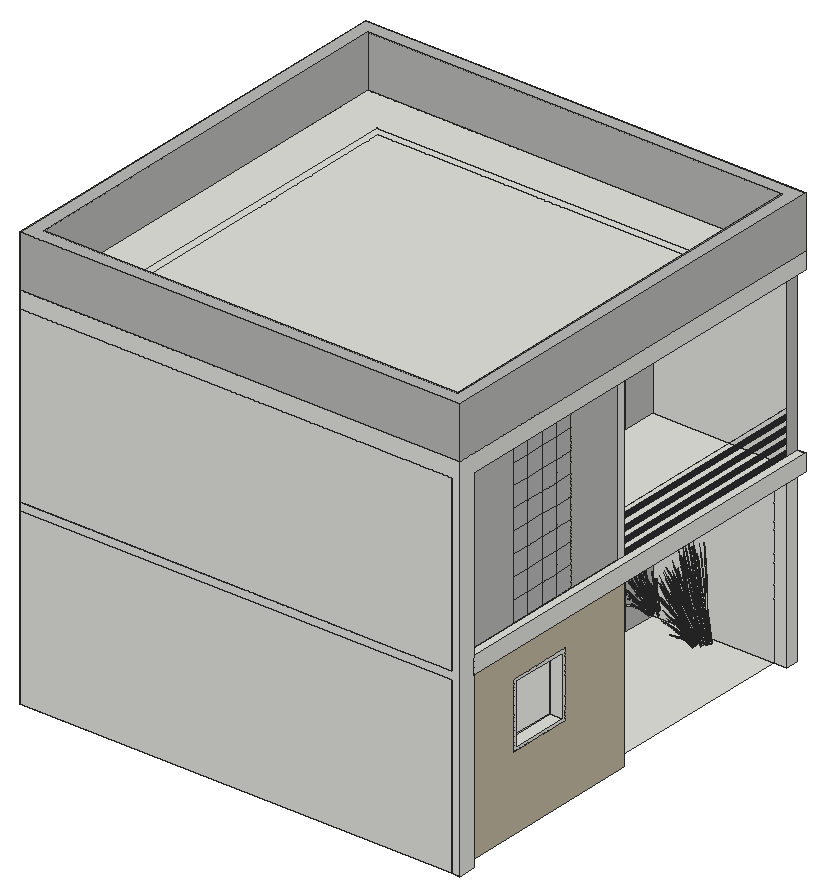
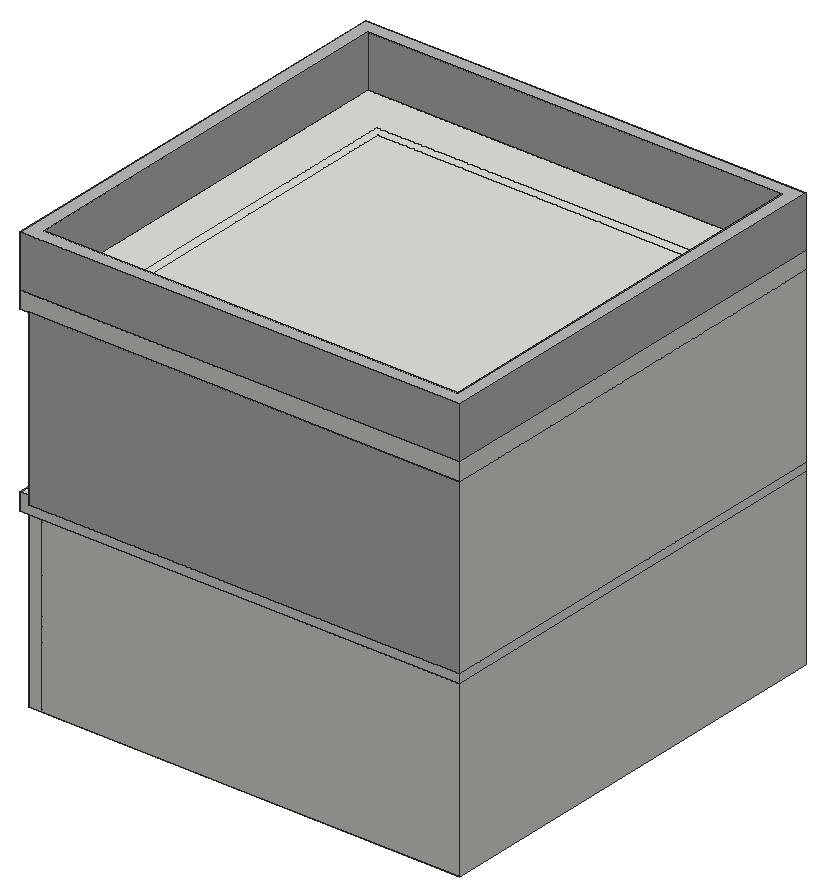
# SketchUp Ruby script. Lengths in inches.
U = 1.inch
M = Sketchup.active_model
def pt(a) = Geom::Point3d.new(a.map { |v| v * U })
def face(e, loops, mat)
  f = e.add_face(loops[0].map { |a| pt(a) })
  loops[1..].each { |l| e.add_face(l.map { |a| pt(a) }).erase! }
  f.material = f.back_material = mat if mat
  f
end
# faces: each face lists its corners as indices into pts; further lists are holes
def faces(e, pts, list, mat = nil) = list.each { |f| face(e, (f[0].is_a?(Array) ? f : [f]).map { |l| l.map { |i| pts[i] } }, mat) }
# xy, xz, yz: faces in a plane at the given z, y or x. An outline is a flat list of corners, or four numbers for a rectangle; further outlines are holes
def ring(l) = l.size == 4 ? [[l[0], l[1]], [l[2], l[1]], [l[2], l[3]], [l[0], l[3]]] : l.each_slice(2).to_a
def flat(e, list, mat, &to3) = list.each { |f| face(e, (f[0].is_a?(Array) ? f : [f]).map { |l| ring(l).map { |u, v| to3.(u, v) } }, mat) }
def xy(e, z, list, mat = nil) = flat(e, list, mat) { |x, y| [x, y, z] }
def xz(e, y, list, mat = nil) = flat(e, list, mat) { |x, z| [x, y, z] }
def yz(e, x, list, mat = nil) = flat(e, list, mat) { |y, z| [x, y, z] }
def lines(e, pts, list) = list.each { |a, b| e.add_line(pt(pts[a]), pt(pts[b])) }
# prism: a flat outline (further loops are holes) pulled along v
def prism(e, loops, v, mat = nil)
  f = face(e, loops, mat); d = Geom::Vector3d.new(v.map { |x| x * U })
  f.pushpull(f.normal.samedirection?(d) ? d.length : -d.length)
end
def box(e, o, s, mat = nil) = prism(e, [[o, [o[0] + s[0], o[1], o[2]], [o[0] + s[0], o[1] + s[1], o[2]], [o[0], o[1] + s[1], o[2]]]], [0, 0, s[2]], mat)
def at(x, y, z, deg = 0) = Geom::Transformation.translation(pt([x, y, z])) * Geom::Transformation.rotation(ORIGIN, Z_AXIS, deg.degrees)
def axes(o, x, y, z) = Geom::Transformation.new([*x, 0, *y, 0, *z, 0, *pt(o).to_a, 1])
def part(name) = M.definitions.add(name)
# library, detail: a bought-in or finely detailed component or shape, given as its bounding box
def library(name, o, s) = part(name).tap { |d| box(d.entities, o, s) }
def detail(e, o, s) = box(e.add_group.entities, o, s)
def put(e, d, t, mat = nil) = e.add_instance(d, t).tap { |i| i.material = mat if mat }
def group(e, t, mat = nil) = e.add_group.tap { |g| g.transformation = t; g.material = mat if mat }.entities
root = M.entities
M.materials.add("Brick_05_1K").color = [195, 185, 161]
M.materials.add("Glass_Basic_01").color = [161, 173, 186]
M.materials["Glass_Basic_01"].alpha = 0.25
M.materials.add("Glass_Mirror_01").color = [185, 185, 185]
M.materials.add("LightPink_Translucent").color = [144, 107, 117]
M.materials["LightPink_Translucent"].alpha = 0.75
M.materials.add("Plywood_01_1K").color = [125, 96, 64]
M.materials.add("ThomThom - Buttons1").color = [48, 49, 53]
M.materials.add("ThomThom - Waistcoat2").color = [186, 186, 184]
M.materials.add("Wood_Veneer_15_1K").color = [103, 69, 45]
c1 = part("blade")
p = [[2.15,0.21,22],[0,0.17,0],[0.09,0.45,0],[2.18,0.31,22],[2.29,0.31,22],[0.38,0.45,0],
  [2.48,0.24,33],[2.49,0.24,33],[2.48,0.22,33]]
faces(c1.entities,p,[[0,1,2,3],[4,5,2,3],[6,3,4,7],[8,0,3,6]])
c2 = part("blade with seeds\#1")
put(c2.entities,c1,at(0,0,0))
c3 = part("seeds")
p = [[0.3,-0.1,1.38],[-0.01,-0.03,1.59],[-0.01,-0.03,0.03],[0.14,-0.07,-0.07],[0.29,-0.03,3],[0.15,0.01,3.11]]
faces(c3.entities,p,[[0,1,2,3],[1,0,4,5]],"LightPink_Translucent")
c4 = part("blade with seeds")
put(c4.entities,c1,at(0,0,0))
put(c4.entities,c3,axes([2.4,0.25,30.99],[1.5799,-0.05474,1.17369],[-0.12525,1.92788,0.29478],[-0.07173,-0.02425,1.56792]))
g1 = group(root,at(0,0,0))
xy(g1,0,[[9,9,291,144],[9,150,291,291]])
g2 = group(g1,at(0,0,0))
xy(g2,0,[[[0,0,0,300,300,300,300,291,207,291,207,150,300,150,300,0],[9,9,291,9,291,144,9,144,9,150,201,150,201,291,9,291]]])
xy(g2,3,[[201,174,207,216],[201,222,207,264]])
xy(g2,53.72,[[291,55.83,300,96.48]])
xy(g2,81,[[201,174,207,216],[201,222,207,264]])
xy(g2,94.93,[[291,55.83,300,96.48]])
xz(g2,0,[[0,0,300,120]])
xz(g2,9,[[9,0,291,120]])
xz(g2,55.83,[[291,53.72,300,94.93]])
xz(g2,96.48,[[291,53.72,300,94.93]])
xz(g2,144,[[9,0,291,120]])
xz(g2,150,[[9,0,201,120],[207,0,300,120]])
xz(g2,174,[[201,3,207,81]])
xz(g2,216,[[201,3,207,81]])
xz(g2,222,[[201,3,207,81]])
xz(g2,264,[[201,3,207,81]])
xz(g2,291,[[9,0,201,120],[201,0,207,120],[207,0,291,120],[291,0,300,120]])
xz(g2,300,[[0,0,291,120],[291,0,300,120]])
yz(g2,0,[[0,0,300,120]])
yz(g2,9,[[9,0,144,120],[144,0,150,120],[150,0,291,120]])
yz(g2,201,[[[150,0,291,120],[222,3,264,81],[174,3,216,81]]])
yz(g2,201,[[174,3,216,81],[222,3,264,81]],"Glass_Basic_01")
yz(g2,207,[[150,0,171,0,171,84,267,84,267,0,291,0,291,120,150,120]],"ThomThom - Waistcoat2")
yz(g2,207,[[[171,0,219,84],[174,3,216,81]],[[219,0,267,84],[222,3,264,81]]],"Wood_Veneer_15_1K")
yz(g2,291,[[[9,0,144,120],[55.83,53.72,96.48,94.93]]])
yz(g2,300,[[291,0,300,120],[[53.83,51.72,98.48,96.93],[55.83,53.72,96.48,94.93]]])
yz(g2,300,[[[0,0,150,120],[53.83,51.72,98.48,96.93]]],"Brick_05_1K")
p = [[207,150,126],[207,150,120]]
lines(g2,p,[[0,1]])
g3 = group(g1,at(0,0,120))
xy(g3,-120,[[300,0,306,12]])
xy(g3,0,[[0,0,0,300,306,300,306,12,300,12,300,0]])
xy(g3,6,[[0,0,300,300]])
xy(g3,12,[[300,12,306,300]])
xy(g3,126,[[0,0,300,12],[0,12,306,300]])
xy(g3,138,[[[9,9,297,291],[39,39,267,261]],[[39,39,267,261],[45,45,261,255]],[45,45,261,255]])
xz(g3,0,[[300,-120,306,-120,306,138,0,138,0,126,300,126,300,6,0,6,0,0,300,0]])
xz(g3,12,[[300,-120,306,0],[300,12,306,126]])
xz(g3,300,[[0,0,0,6,300,6,300,12,306,12,306,0],[0,126,306,138]])
yz(g3,0,[[0,0,300,6],[0,126,300,138]])
yz(g3,300,[[0,-120,12,0],[0,6,0,126,12,126,12,12,300,12,300,6]])
yz(g3,306,[[0,-120,12,-120,12,126,300,126,300,138,0,138],[12,0,300,12]])
g4 = group(g3,at(0,0,138),"ThomThom - Waistcoat2")
prism(g4,[[[306,300,0],[306,0,0],[0,0,0],[0,300,0]],[[297,291,0],[9,291,0],[9,9,0],[297,9,0]]],[0,0,36])
g5 = group(g1,at(0,0,126))
xy(g5,0,[[[0,0,0,300,300,300,300,291,207,291,207,150,201,150,201,291,9,291,9,9,201,9,201,144,9,144,9,150,300,150,300,0],[207,9,291,144]]])
xy(g5,3,[[201,174,207,216],[201,222,207,264]])
xy(g5,81,[[201,174,207,216],[201,222,207,264]])
xy(g5,120,[[[0,0,300,0,300,144,291,144,291,9,207,9,207,291,300,291,300,300,0,300],[9,9,9,291,201,291,201,150,9,150,9,144,201,144,201,9]],[207,144,300,150]])
xz(g5,0,[[0,0,300,120]])
xz(g5,9,[[9,0,201,120],[201,0,207,120],[207,0,291,120]])
xz(g5,144,[[9,0,201,120],[207,0,291,120]])
xz(g5,150,[[9,0,201,120],[207,0,300,36]])
xz(g5,150,[[207,36,300,120]],"ThomThom - Waistcoat2")
xz(g5,174,[[201,3,207,81]])
xz(g5,216,[[201,3,207,81]])
xz(g5,222,[[201,3,207,81]])
xz(g5,264,[[201,3,207,81]])
xz(g5,291,[[9,0,201,120],[207,0,300,120]])
xz(g5,300,[[0,0,300,120]],"ThomThom - Waistcoat2")
yz(g5,0,[[0,0,300,120]])
yz(g5,9,[[9,0,144,120],[144,0,150,120],[150,0,291,120]])
yz(g5,201,[[9,0,144,120],[[150,0,291,120],[222,3,264,81],[174,3,216,81]]])
yz(g5,201,[[174,3,216,81],[222,3,264,81]],"Plywood_01_1K")
yz(g5,207,[[9,0,144,120],[[171,0,219,84],[174,3,216,81]],[[219,0,267,84],[222,3,264,81]]])
yz(g5,207,[[150,0,171,0,171,84,267,84,267,0,291,0,291,120,150,120]],"ThomThom - Waistcoat2")
yz(g5,291,[[9,0,144,120]])
yz(g5,300,[[144,0,150,120],[150,0,291,5.71]])
yz(g5,300,[[53.1875,6,65.8,20.25],[65.8,6,78.41,20.25],[78.41,6,91.03,20.25],[91.03,6,103.64,20.25],[53.1875,20.25,65.8,34.5],
  [65.8,20.25,78.41,34.5],[78.41,20.25,91.03,34.5],[91.03,20.25,103.64,34.5],[53.1875,34.5,65.8,48.75],[65.8,34.5,78.41,48.75],
  [78.41,34.5,91.03,48.75],[91.03,34.5,103.64,48.75],[53.1875,48.75,65.8,63],[65.8,48.75,78.41,63],[78.41,48.75,91.03,63],
  [91.03,48.75,103.64,63],[53.1875,63,65.8,77.25],[65.8,63,78.41,77.25],[78.41,63,91.03,77.25],[91.03,63,103.64,77.25],
  [53.1875,77.25,65.8,91.5],[65.8,77.25,78.41,91.5],[78.41,77.25,91.03,91.5],[91.03,77.25,103.64,91.5],[53.1875,91.5,65.8,105.75],
  [65.8,91.5,78.41,105.75],[78.41,91.5,91.03,105.75],[91.03,91.5,103.64,105.75],[53.1875,105.75,65.8,120],[65.8,105.75,78.41,120],
  [78.41,105.75,91.03,120],[91.03,105.75,103.64,120]],"Glass_Mirror_01")
yz(g5,300,[[150,5.71,291,9.5],[150,13.28,291,17.07],[150,20.86,291,24.64],[150,28.43,291,32.21]],"ThomThom - Buttons1")
yz(g5,300,[[0,0,144,0,144,120,103.64,120,103.64,6,53.1875,6,53.1875,120,0,120],[291,0,300,120]],"ThomThom - Waistcoat2")
p = [[300,150,36],[300,291,36]]
lines(g5,p,[[0,1]])
put(root,c2,axes([216.57,273.84,13.09],[-0.07697,0.17304,1.5897],[-0.85991,0.44448,-0.24285],[-0.23336,-0.29985,0.27078]))
put(root,c2,axes([218.64,273.875,15.96],[-0.89213,0.297,-0.46065],[-0.15606,-1.12475,-0.35681],[-0.23962,-0.32232,0.88141]))
put(root,c2,axes([219,273.85,16.23],[-0.77091,-0.6039,-0.64046],[0.54787,-1.05824,0.07729],[-0.27931,-0.36058,0.906]))
put(root,c2,axes([219.28,273.34,16.28],[-0.53874,1.06944,-0.10962],[-0.78019,-0.61612,-0.60845],[-0.2712,-0.30214,0.92453]))
put(root,c2,axes([218.29,272.97,14.08],[-0.02894,0.41302,1.28914],[-0.77632,0.42312,-0.27724],[-0.21961,-0.50739,0.55117]))
put(root,c2,axes([219.04,270.71,15.98],[-0.00742,0.151,1.59908],[-0.79509,0.62706,-0.1511],[-0.26143,-0.25182,0.28298]))
put(root,c2,axes([216.86,272.49,14.23],[0.49736,0.38508,1.03545],[-0.66822,0.331,0.76078],[-0.16744,-0.31805,0.22807]))
put(root,c2,axes([218.73,273.05,15.82],[-0.13963,-1.00636,-0.31925],[0.79822,-0.26574,0.41216],[-0.2144,-0.28839,0.78863]))
put(root,c2,axes([218.9,273.18,16.01],[0.89921,-0.28673,0.43274],[0.15606,1.12475,0.35681],[-0.21148,-0.33149,0.89544]))
put(root,c2,axes([219.08,272.95,16],[0.4109,-0.79368,0.05797],[0.58514,0.46209,0.45634],[-0.18917,-0.25446,0.69585]))
put(root,c2,axes([219.99,270.14,15.99],[-0.14882,-0.16043,1.57709],[-0.91289,0.20534,-0.24942],[-0.17308,-0.40254,0.12648]))
put(root,c2,axes([217,275.05,13.88],[-0.97904,-0.72283,0],[0.54599,-1.20931,-0.46523],[0.12435,-0.27543,1.47583]))
put(root,c2,axes([221.38,273.3,16.28],[-0.88471,0.5817,-0.10962],[-0.43476,-1.03242,-0.60845],[-0.11673,-0.43507,0.92453]))
put(root,c2,axes([220.62,273.35,15.96],[-0.88873,-0.31321,-0.46065],[0.30463,-1.07385,-0.35681],[-0.08149,-0.43235,0.88141]))
put(root,c2,axes([220.87,272.21,13.53],[0.11725,0.74462,1.27635],[-0.9333,0.11852,0.07306],[-0.14126,-0.52153,0.72629]))
put(root,c2,axes([220.04,270.85,13.78],[-0.62476,0.71677,-0.05849],[-0.57245,-0.78502,-0.26518],[-0.0403,-0.22243,0.87466]))
put(root,c2,axes([220.94,273.56,16.23],[-0.4315,-1.0159,-0.64046],[0.88824,-0.56616,0.07729],[-0.1009,-0.49086,0.906]))
put(root,c2,axes([221.11,273.71,16.29],[-0.27256,0.96081,0.31925],[-0.79518,-0.28024,-0.41216],[-0.07291,-0.38684,0.78863]))
put(root,c2,axes([220.26,271.39,13.09],[-0.14833,0.06042,1.5897],[-0.86768,-0.41907,-0.24285],[-0.01248,-0.42273,0.27078]))
put(root,c2,axes([217.59,274.39,13.56],[0.48852,-1.08202,-0.44759],[0.87598,0.64674,0],[0.11126,-0.24644,1.41987]))
put(root,c2,axes([221.02,272.69,15.82],[0.27256,-0.96081,-0.31925],[0.79518,0.28024,0.41216],[-0.07291,-0.38684,0.78863]))
put(root,c2,axes([220.04,275.3125,15.23],[0.02213,0.47954,1.54493],[-0.95907,-0.31812,0.12492],[0.05932,-0.68338,0.66044]))
put(root,c2,axes([221.36,272.84,16],[0.66618,-0.42462,0.05797],[0.32607,0.77431,0.45634],[-0.06434,-0.34133,0.69585]))
put(root,c2,axes([221.12,272.92,16.01],[0.89085,0.32663,0.43274],[-0.30463,1.07385,0.35681],[-0.05354,-0.4223,0.89544]))
put(root,c2,axes([221.1875,270.66,14.23],[0.1613,0.71432,1.03545],[-0.66662,-0.33623,0.76078],[0.04561,-0.37895,0.22807]))
put(root,c2,axes([219.46,275.97,13.6],[0.16018,-1.20264,-0.5621],[0.98808,0.25378,-0.14753],[0.11973,-0.3589,1.24074]))
put(root,c2,axes([224.01,270.99,15.98],[-0.08553,0.10454,1.59908],[-0.91687,-0.22868,-0.1511],[-0.05858,-0.41178,0.28298]))
put(root,c2,axes([223.24,271.9,15.28],[-0.82131,0.22128,-0.03148],[-0.18882,-1.04586,-0.14272],[0.05207,-0.2184,0.47074]))
put(root,c2,axes([223.22,274.61,16.28],[-0.99362,-0.0619,-0.10962],[0.02716,-1.17208,-0.60845],[0.06902,-0.45141,0.92453]))
put(root,c2,axes([222.83,274.79,16.29],[-0.61172,0.65782,0.31925],[-0.57907,-0.75112,-0.41216],[0.08811,-0.38163,0.78863]))
put(root,c2,axes([222.25,272,14.08],[-0.2403,0.27843,1.28914],[-0.79492,-0.36227,-0.27724],[0.10768,-0.56334,0.55117]))
put(root,c2,axes([222.62,273.59,15.99],[-0.01652,-0.24801,1.57709],[-0.75906,-0.68026,-0.24942],[0.1002,-0.44114,0.12648]))
put(root,c2,axes([222.74,274.55,16.23],[0.02352,-1.1557,-0.64046],[0.99061,0.07762,0.07729],[0.10454,-0.48961,0.906]))
put(root,c2,axes([223.15,273.86,15.82],[0.61172,-0.65782,-0.31925],[0.57907,0.75112,0.41216],[0.08811,-0.38163,0.78863]))
put(root,c2,axes([223.38,274.19,16],[0.74296,0.05822,0.05797],[-0.02037,0.87906,0.45634],[0.07774,-0.33673,0.69585]))
put(root,c2,axes([223.14,274.11,16.01],[0.64379,0.85247,0.43274],[-0.68369,0.73521,0.35681],[0.11875,-0.39995,0.89544]))
put(root,c2,axes([221.58,276.22,15.23],[-0.16834,0.42944,1.54493],[-0.70619,-0.88871,0.12492],[0.31858,-0.5539,0.66044]))
put(root,c2,axes([224.54,274.45,13.09],[-0.14106,-0.08423,1.5897],[-0.41543,-1.06044,-0.24285],[0.21501,-0.3215,0.27078]))
put(root,c2,axes([223.88,276.1,15.96],[-0.23225,-1.14083,-0.46065],[0.87956,-0.19957,-0.35681],[0.25205,-0.30642,0.88141]))
put(root,c4,axes([260.33,260.75,16.11],[0.50831,-0.02346,1.71376],[-0.33721,1.01661,0.13857],[-0.72439,-0.06288,0.73262]))
put(root,c4,axes([260.54,262.54,16.11],[0.42521,-0.21906,1.71376],[0.35798,1.01226,0.13857],[-0.66754,0.22878,0.73262]))
put(root,c4,axes([259.22,264.27,14.83],[0.42589,0.08502,1.43002],[0.2745,0.86839,-0.30754],[-0.57851,0.16255,0.61141]))
put(root,c4,axes([262.98,261.49,15.58],[0.34834,-0.14982,1.77064],[0.12012,1.04605,0.13857],[-0.75452,0.1388,0.63284]))
put(root,c4,axes([259.24,262.1875,16.95],[-0.20012,0.13446,1.74944],[0.01702,0.98243,-0.27667],[-0.45871,0.12776,0.14031]))
put(root,c4,axes([261.85,259.81,17.22],[-1.22504,-0.02494,-0.71045],[0.08228,-1.05005,0.08574],[-0.51899,-0.11081,1.00501]))
put(root,c4,axes([260.86,260.07,14.83],[0.23927,0.28834,1.43002],[-0.55135,0.78376,-0.30754],[-0.56612,-0.18733,0.61141]))
put(root,c4,axes([259.88,261.63,16.76],[-1.01846,-0.28891,-0.35414],[0.29705,-0.84289,0.4572],[-0.41005,0.07729,0.87481]))
put(root,c4,axes([261.29,259.125,16.11],[0.45521,0.17844,1.71376],[-0.94204,0.74856,0.13857],[-0.58713,-0.33769,0.73262]))
put(root,c4,axes([257.01,263.18,16.95],[0.1564,0.02778,1.77383],[0.48382,0.91506,-0.16761],[-0.32016,0.24017,0.31391]))
put(root,c4,axes([260.58,262.06,16.92],[-0.332,0.94205,-0.51099],[-1.13828,-0.3229,-0.3958],[-0.45829,0.08638,0.97773]))
put(root,c4,axes([261.44,260.02,16.92],[-0.88986,0.68603,-0.51099],[-0.77932,-0.72471,-0.3958],[-0.45212,-0.10438,0.97773]))
put(root,c4,axes([260.01,262,13.73],[0.03108,0.16322,1.76342],[-0.62654,0.85237,-0.26939],[-0.44504,-0.04296,0.30037]))
put(root,c4,axes([260.1875,258.1,16.95],[0.09085,0.10335,1.77383],[-0.43798,0.92907,-0.16761],[-0.44357,0.00672,0.31391]))
put(root,c4,axes([258.33,266.09,15],[0.51072,-0.46938,1.1486],[0.20153,0.74307,0.84392],[-0.36908,0.13305,0.25299]))
put(root,c4,axes([261.2,257.48,16.95],[-0.26368,-0.00731,1.74944],[-0.83946,0.73103,-0.27667],[-0.44791,-0.14937,0.14031]))
put(root,c4,axes([260.12,261.52,16.97],[0.34623,-0.9443,0.48003],[1.13828,0.3229,0.3958],[-0.44763,0.05675,0.9933]))
put(root,c4,axes([260.52,261.25,17.27],[0.6166,0.93779,-0.1216],[-1.09436,0.46085,-0.67495],[-0.46117,0.12373,1.02557]))
put(root,c4,axes([261.91,259.3,17.27],[-0.06562,1.05324,-0.1216],[-1.2424,-0.02879,-0.67495],[-0.4785,-0.07316,1.02557]))
put(root,c4,axes([261.11,259.38,16.76],[-0.69728,-0.64842,-0.35414],[0.79619,-0.61382,0.4572],[-0.40453,-0.09339,0.87481]))
put(root,c4,axes([260.03,261.27,16.97],[-0.4501,-0.70615,0.0643],[0.82077,-0.34564,0.50621],[-0.36181,0.0682,0.77189]))
put(root,c4,axes([260.25,264.06,16.76],[-1.06674,0.14801,-0.35414],[-0.28168,-0.84611,0.4572],[-0.30569,0.22726,0.87481]))
put(root,c4,axes([259.4375,260.93,15],[0.78239,-0.07411,1.1486],[-0.49629,0.65296,0.84392],[-0.38663,-0.09795,0.25299]))
put(root,c4,axes([260.39,263.875,16.97],[-0.30393,-0.95317,0.48003],[1.19224,-0.16542,0.3958],[-0.35138,0.22417,0.9933]))
put(root,c4,axes([261.01,259.13,17.33],[1.01205,-0.7643,0.53763],[0.87284,0.81167,0.4433],[-0.47482,-0.14098,1.11249]))
put(root,c4,axes([260.16,263.69,16.97],[-0.8413,-0.43556,0.0643],[0.48981,-0.62025,0.50621],[-0.26973,0.20053,0.77189]))
put(root,c4,axes([260.95,261.54,17.29],[1.01846,0.28891,0.35414],[-0.29705,0.84289,-0.4572],[-0.41005,0.07729,0.87481]))
put(root,c4,axes([261.47,259.13,16.97],[0.06171,-0.78753,0.0643],[0.9318,0.02159,0.50621],[-0.35694,-0.08241,0.77189]))
put(root,c4,axes([264.11,263.48,14.3],[-1.27479,-0.1698,-0.62353],[0.26901,-1.04736,-0.16365],[-0.38043,-0.12691,1.37633]))
put(root,c4,axes([264.34,257.77,17.67],[-0.81789,0.99285,-0.13619],[-1.18445,-0.572,-0.75594],[-0.41173,-0.28051,1.14864]))
put(root,c4,axes([262.1,259.72,17.29],[0.69728,0.64842,0.35414],[-0.79619,0.61382,-0.4572],[-0.40453,-0.09339,0.87481]))
put(root,c4,axes([263.98,258.57,17.22],[-1.04497,-0.50058,-0.71045],[0.74264,-0.8772,0.08574],[-0.3786,-0.29889,1.00501]))
put(root,c4,axes([263.49,258.6,16.92],[-1.20928,0.24619,-0.51099],[-0.21154,-0.93233,-0.3958],[-0.32481,-0.26718,0.97773]))
put(root,c4,axes([262.43,265.46,14.25],[-1.14694,-0.51783,-0.49651],[0.68554,-0.92854,0],[-0.26122,-0.11794,1.57504]))
put(root,c4,axes([261.93,257.75,13.73],[-0.11871,0.13643,1.76342],[-1.19964,0.29415,-0.26939],[-0.2898,-0.26759,0.30037]))
put(root,c4,axes([260.57,263.48,17.27],[1.1336,0.57106,-0.1216],[-0.65308,0.827,-0.67495],[-0.32027,0.28747,1.02557]))
put(root,c4,axes([263.13,266.09,14.61],[-0.7662,1.03778,0],[-1.28187,-0.57875,-0.51607],[-0.29196,-0.13181,1.63711]))
put(root,c4,axes([258.7,265.96,17.88],[1.08141,0.27645,-0.06488],[-0.33265,0.85086,-0.29416],[-0.17688,0.12919,0.97024]))
put(root,c4,axes([261.125,263.56,17.29],[1.06674,-0.14801,0.35414],[0.28168,0.84611,-0.4572],[-0.30569,0.22726,0.87481]))
put(root,c4,axes([261.18,258.27,14.36],[-0.35352,0.84566,-0.03893],[-1.08806,-0.26014,-0.17649],[-0.1652,-0.13832,0.58215]))
put(root,c4,axes([264.02,255.41,16.95],[-0.02286,0.12414,1.77383],[-1.12758,0.45052,-0.16761],[-0.33182,-0.23029,0.31391]))
put(root,c4,axes([262.81,257.21,14.83],[-0.07421,0.33879,1.43002],[-1.08488,0.28361,-0.30754],[-0.25359,-0.4379,0.61141]))
put(root,c4,axes([263.16,258.09,16.11],[0.28013,0.33252,1.71376],[-1.29445,0.27994,0.13857],[-0.29256,-0.52202,0.73262]))
put(root,c4,axes([265.55,263.63,14.9],[-1.23732,0.68758,-0.29095],[-0.8228,-0.97154,-0.50002],[-0.30528,-0.09867,1.59708]))
put(root,c4,axes([263.62,257.91,16.76],[-0.18927,-0.83419,-0.35414],[1.08199,-0.22027,0.4572],[-0.29062,-0.23905,0.87481]))
put(root,c4,axes([260.6,262.13,14.61],[-1.53239,0,0],[0,-1.1575,-0.51607],[0,-0.26363,1.63711]))
put(root,c4,axes([262.75,265.07,14.26],[-0.28787,-0.90242,-0.30978],[1.14332,-0.25625,0.30978],[-0.23049,-0.10406,1.38974]))
put(root,c4,axes([266.375,264.38,14.3],[-0.82544,0.77843,-0.62353],[-1.0254,-0.70586,-0.16365],[-0.33076,0.19418,1.37633]))
put(root,c4,axes([264.26,258.59,17.29],[0.18927,0.83419,0.35414],[-1.08199,0.22027,-0.4572],[-0.29062,-0.23905,0.87481]))
put(root,c4,axes([261.79,261.83,14.57],[-1.1399,0.87071,0.30756],[-1.1406,-0.86155,-0.36492],[-0.03981,-0.24727,1.64885]))
put(root,c4,axes([266.48,264.24,15.5625],[1.05902,0.41762,1.51261],[-1.03748,0.89969,0.59816],[-0.46471,-0.53324,1.26806]))
put(root,c4,axes([262.4375,256.66,15],[0.63926,0.36046,1.1486],[-0.93099,0.21668,0.84392],[-0.1992,-0.27702,0.25299]))
put(root,c4,axes([266.94,263.95,14.7],[-1.19666,-0.83357,-0.25192],[1.00694,-0.93603,0.5513],[-0.32224,0.09751,1.68216]))
put(root,c4,axes([264.77,263.15,14.45],[-0.73619,-0.86927,-0.44739],[1.11511,-0.61213,0.21531],[-0.23824,-0.10756,1.43643]))
put(root,c4,axes([263.77,257.61,17.33],[1.36515,-0.26619,0.53763],[0.23692,1.04421,0.4433],[-0.32106,-0.30775,1.11249]))
put(root,c4,axes([266.34,263.77,14.45],[-1.33077,0.06393,-0.44739],[-0.12035,-1.06125,0.21531],[-0.23824,0.10756,1.43643]))
put(root,c4,axes([264.09,257.83,16.97],[0.55698,-0.6579,0.0643],[0.79316,0.38303,0.50621],[-0.25643,-0.21093,0.77189]))
put(root,c4,axes([263.79,265.54,14.71],[1.14694,0.51783,0.49651],[-0.68554,0.92854,0],[-0.26122,-0.11794,1.57504]))
put(root,c4,axes([264.875,263.64,14.68],[0.32481,-1.2272,-0.23429],[1.54007,0.21392,0.51271],[-0.26911,-0.16947,1.5644]))
put(root,c4,axes([265.43,263.93,14.85],[-0.23642,0.92427,0.1448],[-1.15506,-0.16044,-0.41347],[-0.21021,-0.09491,1.26744]))
put(root,c4,axes([265.3,255.88,16.95],[-0.18744,-0.14521,1.74944],[-1.25089,0.09206,-0.27667],[-0.19964,-0.34731,0.14031]))
put(root,c4,axes([267.73,266.51,14.25],[-1.14694,0.51783,-0.49651],[-0.68554,-0.92854,0],[-0.26122,0.11794,1.57504]))
put(root,c4,axes([260.94,261.35,14.25],[0,-1.03566,-0.49651],[1.37109,0,0],[0,-0.23588,1.57504]))
put(root,c4,axes([261.53,262.31,14.71],[0,1.03566,0.49651],[-1.37109,0,0],[0,-0.23588,1.57504]))
put(root,c4,axes([267.81,266.23,14.43],[-0.75665,-1.04141,-0.05142],[1.28187,-0.57875,0.51607],[-0.31588,0.09915,1.6363]))
put(root,c4,axes([267.46,266.1,14.26],[-1.14332,-0.25625,-0.30978],[0.28787,-0.90242,0.30978],[-0.23049,0.10406,1.38974]))
put(root,c4,axes([264.53,262.55,14.9],[-1.38012,-0.49416,-0.29095],[0.66454,-1.04299,-0.50002],[-0.04337,-0.25608,1.59708]))
put(root,c4,axes([267.27,263.48,14.9],[0.1428,1.18174,-0.29095],[-1.48733,0.07145,-0.50002],[-0.26191,0.15741,1.59708]))
put(root,c4,axes([263.91,261.5,14.33],[-0.50328,-1.06202,-0.69835],[1.44974,-0.38248,-0.18329],[-0.05563,-0.35963,1.54149]))
put(root,c4,axes([267.21,258.12,17.27],[-1.19922,0.48218,-0.1216],[-0.58932,-0.85579,-0.67495],[-0.15822,-0.36063,1.02557]))
